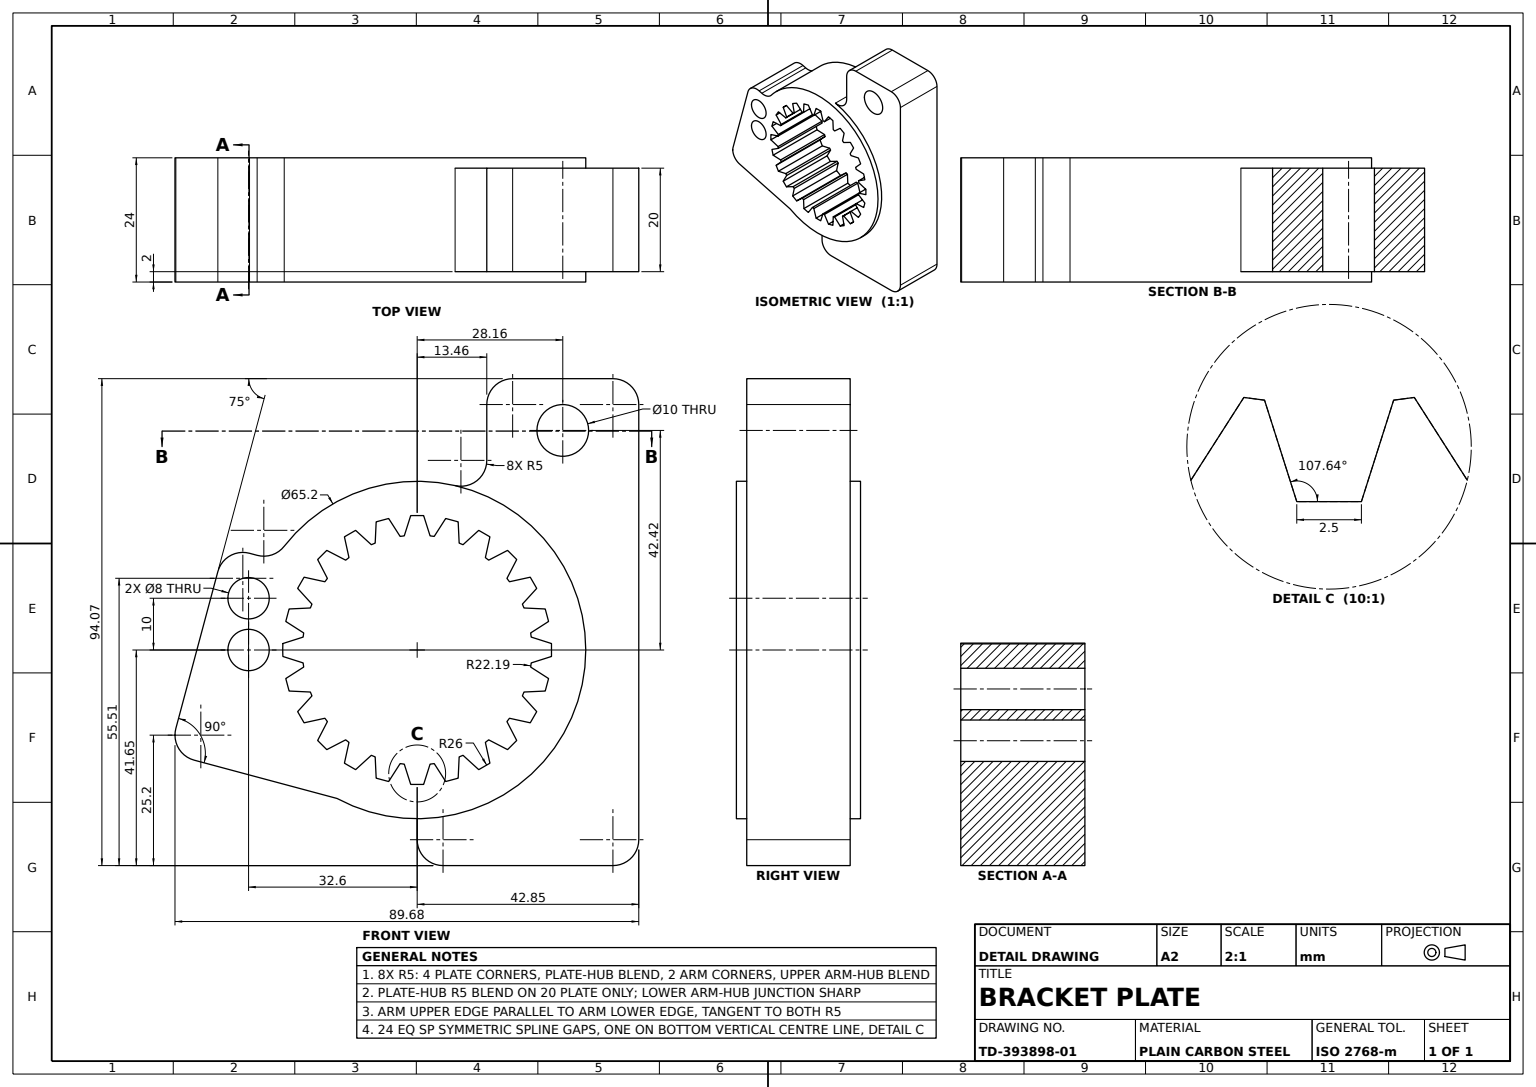
solid
v1 (-20.651843,-8.117725,-12)
v2 (-20.343157,-8.86296,-12)
e1 v1 v2 CIRCLE(AX(P(0,0,-12),D(0,0,1),D(1,0,0)),22.19)
v3 (-20.651843,-8.117725,12)
e2 v3 v1 LINE
v4 (-20.343157,-8.86296,12)
e3 v3 v4 CIRCLE(AX(P(0,0,12),D(0,0,1),D(1,0,0)),22.19)
e4 v4 v2 LINE
face CYL(AX(P(0,0,12),D(0,0,-1),D(-1,0,0)),22.19) rev [-e1 -e2 e3 e4]
v5 (7.335,31.764096,10)
v6 (0,-32.6,10)
e5 v5 v6 CIRCLE(AX(P(0,0,10),D(0,0,-1),D(1,0,0)),32.6)
v7 (0,-36.65,10)
e6 v6 v7 LINE
v8 (5,-41.65,10)
e7 v7 v8 CIRCLE(AX(P(5,-36.65,10),D(0,0,1),D(-1,0,0)),5)
v9 (37.85,-41.65,10)
e8 v8 v9 LINE
v10 (42.85,-36.65,10)
e9 v9 v10 CIRCLE(AX(P(37.85,-36.65,10),D(0,0,1),D(-1,0,0)),5)
v11 (42.85,47.42,10)
e10 v10 v11 LINE
v12 (37.85,52.42,10)
e11 v11 v12 CIRCLE(AX(P(37.85,47.42,10),D(0,0,1),D(-1,0,0)),5)
v13 (18.46,52.42,10)
e12 v12 v13 LINE
v14 (13.46,47.42,10)
e13 v13 v14 CIRCLE(AX(P(18.46,47.42,10),D(0,0,1),D(-1,0,0)),5)
v15 (13.46,36.63589,10)
e14 v14 v15 LINE
e15 v15 v5 CIRCLE(AX(P(8.46,36.63589,10),D(0,0,-1),D(1,0,0)),5)
v16 (33.155,42.42,10)
v17 (23.155,42.42,10)
e16 v16 v17 CIRCLE(AX(P(28.155,42.42,10),D(0,0,1),D(1,0,0)),5)
e17 v17 v16 CIRCLE(AX(P(28.155,42.42,10),D(0,0,1),D(1,0,0)),5)
face PLANE(AX(P(37.85,-36.65,10),D(0,0,-1),D(-1,0,0))) rev [e5 e6 e7 e8 e9 e10 e11 e12 e13 e14 e15] [-e16 -e17]
v18 (25.408478,5.51446,12)
v19 (25.408478,5.51446,-12)
e18 v18 v19 LINE
v20 (21.943884,3.295765,-12)
e19 v20 v19 LINE
v21 (21.943884,3.295765,12)
e20 v21 v20 LINE
e21 v21 v18 LINE
face PLANE(AX(P(4.885198,-7.628462,12),D(-0.539287232,0.842121892,0),D(-0.842121892,-0.539287232,0))) [e18 -e19 -e20 e21]
v22 (-2.49603,22.049171,12)
v23 (-3.295765,21.943884,12)
e22 v22 v23 CIRCLE(AX(P(0,0,12),D(0,0,1),D(1,0,0)),22.19)
v24 (-3.295765,21.943884,-12)
e23 v23 v24 LINE
v25 (-2.49603,22.049171,-12)
e24 v25 v24 CIRCLE(AX(P(0,0,-12),D(0,0,1),D(1,0,0)),22.19)
e25 v22 v25 LINE
face CYL(AX(P(0,0,12),D(0,0,-1),D(-1,0,0)),22.19) rev [e22 e23 -e24 -e25]
v26 (1.249639,25.969952,12)
v27 (1.249639,25.969952,-12)
e26 v26 v27 LINE
v28 (2.49603,22.049171,-12)
e27 v28 v27 LINE
v29 (2.49603,22.049171,12)
e28 v29 v28 LINE
e29 v29 v26 LINE
face PLANE(AX(P(8.632911,2.744348,12),D(-0.953005091,-0.302954281,0),D(0.302954281,-0.953005091,0))) [e26 -e27 -e28 e29]
v30 (-1.249639,25.969952,-12)
e30 v27 v30 CIRCLE(AX(P(0,0,-12),D(0,0,1),D(1,0,0)),26)
v31 (-1.249639,25.969952,12)
e31 v26 v31 CIRCLE(AX(P(0,0,12),D(0,0,1),D(1,0,0)),26)
e32 v31 v30 LINE
face CYL(AX(P(0,0,12),D(0,0,-1),D(-1,0,0)),26) rev [-e30 -e26 e31 e32]
v32 (-21.865819,14.067195,12)
v33 (-21.865819,14.067195,-12)
e33 v32 v33 LINE
v34 (-17.847127,13.186211,-12)
e34 v34 v33 LINE
v35 (-17.847127,13.186211,12)
e35 v35 v34 LINE
e36 v35 v32 LINE
face PLANE(AX(P(1.939781,8.848494,12),D(-0.214136442,-0.976803759,0),D(0.976803759,-0.214136442,0))) [e33 -e34 -e35 e36]
v36 (20.343157,-8.86296,12)
v37 (20.651843,-8.117725,12)
e37 v36 v37 CIRCLE(AX(P(0,0,12),D(0,0,1),D(1,0,0)),22.19)
v38 (20.651843,-8.117725,-12)
e38 v37 v38 LINE
v39 (20.343157,-8.86296,-12)
e39 v39 v38 CIRCLE(AX(P(0,0,-12),D(0,0,1),D(1,0,0)),22.19)
e40 v36 v39 LINE
face CYL(AX(P(0,0,12),D(0,0,-1),D(-1,0,0)),22.19) rev [e37 e38 -e39 -e40]
v40 (33.155,42.42,-10)
e41 v40 v16 LINE
v41 (23.155,42.42,-10)
e42 v41 v40 CIRCLE(AX(P(28.155,42.42,-10),D(0,0,1),D(1,0,0)),5)
e43 v41 v17 LINE
face CYL(AX(P(28.155,42.42,-10),D(0,0,1),D(1,0,0)),5) rev [e17 -e41 -e42 e43]
v42 (-26,0,12)
v43 (-26,0,-12)
e44 v42 v43 LINE
v44 (-25.969952,1.249639,-12)
e45 v44 v43 CIRCLE(AX(P(0,0,-12),D(0,0,1),D(1,0,0)),26)
v45 (-25.969952,1.249639,12)
e46 v45 v44 LINE
e47 v45 v42 CIRCLE(AX(P(0,0,12),D(0,0,1),D(1,0,0)),26)
face CYL(AX(P(0,0,12),D(0,0,-1),D(-1,0,0)),26) rev [e44 -e45 -e46 e47]
v46 (-17.356078,13.826158,12)
e48 v46 v35 CIRCLE(AX(P(0,0,12),D(0,0,1),D(1,0,0)),22.19)
v47 (-17.356078,13.826158,-12)
e49 v47 v34 CIRCLE(AX(P(0,0,-12),D(0,0,1),D(1,0,0)),22.19)
e50 v46 v47 LINE
face CYL(AX(P(0,0,12),D(0,0,-1),D(-1,0,0)),22.19) rev [e48 e35 -e49 -e50]
v48 (-43.125337,-21.279101,-12)
v49 (-15.4932,-28.683109,-12)
e51 v48 v49 LINE
v50 (-15.4932,-28.683109,12)
e52 v50 v49 LINE
v51 (-43.125337,-21.279101,12)
e53 v51 v50 LINE
e54 v51 v48 LINE
face PLANE(AX(P(-47.954966,-19.985005,12),D(0.258819045,0.965925826,0),D(-0.965925826,0.258819045,0))) rev [e51 -e52 -e53 e54]
v52 (-38.540423,15.150547,-12)
v53 (-46.660871,-15.155376,-12)
e55 v52 v53 LINE
v54 (-46.660871,-15.155376,12)
e56 v53 v54 LINE
v55 (-38.540423,15.150547,12)
e57 v55 v54 LINE
e58 v55 v52 LINE
face PLANE(AX(P(-37.246328,19.980176,12),D(0.965925826,-0.258819045,0),D(0.258819045,0.965925826,0))) rev [e55 e56 -e57 e58]
v56 (25.408478,-5.51446,12)
v57 (25.408478,-5.51446,-12)
e59 v56 v57 LINE
v58 (21.943884,-3.295765,12)
e60 v58 v56 LINE
v59 (21.943884,-3.295765,-12)
e61 v58 v59 LINE
e62 v59 v57 LINE
face PLANE(AX(P(4.885198,7.628462,12),D(0.539287232,0.842121892,0),D(-0.842121892,0.539287232,0))) rev [-e59 -e60 e61 e62]
v60 (-46.831242,-16.449471,12)
v61 (-46.831242,-16.449471,-12)
e63 v60 v61 LINE
e64 v54 v60 CIRCLE(AX(P(-41.831242,-16.449471,12),D(0,0,1),D(1,0,0)),5)
e65 v61 v53 CIRCLE(AX(P(-41.831242,-16.449471,-12),D(0,0,-1),D(1,0,0)),5)
face CYL(AX(P(-41.831242,-16.449471,12),D(0,0,-1),D(-1,0,0)),5) [-e63 -e64 -e56 -e65]
v62 (3.295765,-21.943884,12)
v63 (3.295765,-21.943884,-12)
e66 v62 v63 LINE
v64 (2.49603,-22.049171,-12)
e67 v64 v63 CIRCLE(AX(P(0,0,-12),D(0,0,1),D(1,0,0)),22.19)
v65 (2.49603,-22.049171,12)
e68 v65 v64 LINE
e69 v65 v62 CIRCLE(AX(P(0,0,12),D(0,0,1),D(1,0,0)),22.19)
face CYL(AX(P(0,0,12),D(0,0,-1),D(-1,0,0)),22.19) rev [e66 -e67 -e68 e69]
v66 (8.86296,20.343157,-12)
v67 (11.902757,23.115457,-12)
e70 v66 v67 LINE
v68 (11.902757,23.115457,12)
e71 v68 v67 LINE
v69 (8.86296,20.343157,12)
e72 v69 v68 LINE
e73 v69 v66 LINE
face PLANE(AX(P(-6.104147,6.693131,12),D(-0.673849478,0.738868649,0),D(-0.738868649,-0.673849478,0))) rev [e70 -e71 -e72 e73]
v70 (20.343157,8.86296,12)
v71 (20.343157,8.86296,-12)
e74 v70 v71 LINE
v72 (23.115457,11.902757,12)
e75 v70 v72 LINE
v73 (23.115457,11.902757,-12)
e76 v72 v73 LINE
e77 v71 v73 LINE
face PLANE(AX(P(6.693131,-6.104147,12),D(-0.738868649,0.673849478,0),D(-0.673849478,-0.738868649,0))) [-e74 e75 e76 -e77]
v74 (-1.249639,-25.969952,12)
v75 (1.249639,-25.969952,12)
e78 v74 v75 CIRCLE(AX(P(0,0,12),D(0,0,1),D(1,0,0)),26)
v76 (1.249639,-25.969952,-12)
e79 v75 v76 LINE
v77 (-1.249639,-25.969952,-12)
e80 v77 v76 CIRCLE(AX(P(0,0,-12),D(0,0,1),D(1,0,0)),26)
e81 v74 v77 LINE
face CYL(AX(P(0,0,12),D(0,0,-1),D(-1,0,0)),26) rev [e78 e79 -e80 -e81]
v78 (37.85,-41.65,-10)
e82 v9 v78 LINE
v79 (42.85,-36.65,-10)
e83 v78 v79 CIRCLE(AX(P(37.85,-36.65,-10),D(0,0,1),D(-1,0,0)),5)
e84 v10 v79 LINE
face CYL(AX(P(37.85,-36.65,10),D(0,0,-1),D(-1,0,0)),5) [e82 e83 -e84 -e9]
v80 (-14.067195,-21.865819,12)
v81 (-14.067195,-21.865819,-12)
e85 v80 v81 LINE
v82 (-11.902757,-23.115457,12)
e86 v80 v82 CIRCLE(AX(P(0,0,12),D(0,0,1),D(1,0,0)),26)
v83 (-11.902757,-23.115457,-12)
e87 v82 v83 LINE
e88 v81 v83 CIRCLE(AX(P(0,0,-12),D(0,0,1),D(1,0,0)),26)
face CYL(AX(P(0,0,12),D(0,0,-1),D(-1,0,0)),26) rev [-e85 e86 e87 -e88]
v84 (-24.761617,-7.928577,-12)
e89 v1 v84 LINE
v85 (-24.761617,-7.928577,12)
e90 v85 v84 LINE
e91 v3 v85 LINE
face PLANE(AX(P(-0.416475,-9.049041,12),D(-0.045975497,-0.998942568,0),D(0.998942568,-0.045975497,0))) rev [e89 -e90 -e91 e2]
v86 (18.46,52.42,-10)
v87 (13.46,47.42,-10)
e92 v86 v87 CIRCLE(AX(P(18.46,47.42,-10),D(0,0,1),D(-1,0,0)),5)
e93 v14 v87 LINE
e94 v13 v86 LINE
face CYL(AX(P(18.46,47.42,10),D(0,0,-1),D(-1,0,0)),5) [e92 -e93 -e13 e94]
v88 (13.186211,-17.847127,-12)
v89 (13.826158,-17.356078,-12)
e95 v88 v89 CIRCLE(AX(P(0,0,-12),D(0,0,1),D(1,0,0)),22.19)
v90 (13.186211,-17.847127,12)
e96 v90 v88 LINE
v91 (13.826158,-17.356078,12)
e97 v90 v91 CIRCLE(AX(P(0,0,12),D(0,0,1),D(1,0,0)),22.19)
e98 v91 v89 LINE
face CYL(AX(P(0,0,12),D(0,0,-1),D(-1,0,0)),22.19) rev [-e95 -e96 e97 e98]
v92 (37.85,52.42,-10)
e99 v92 v86 LINE
e100 v12 v92 LINE
face PLANE(AX(P(37.85,52.42,10),D(0,-1,0),D(0,0,-1))) rev [e99 -e94 -e12 e100]
v93 (-28.6,10,-12)
v94 (-28.6,10,12)
e101 v93 v94 LINE
v95 (-36.6,10,12)
e102 v94 v95 CIRCLE(AX(P(-32.6,10,12),D(0,0,1),D(1,0,0)),4)
v96 (-36.6,10,-12)
e103 v96 v95 LINE
e104 v93 v96 CIRCLE(AX(P(-32.6,10,-12),D(0,0,1),D(1,0,0)),4)
face CYL(AX(P(-32.6,10,-12),D(0,0,1),D(1,0,0)),4) rev [e101 e102 -e103 -e104]
v97 (-17.847127,-13.186211,12)
v98 (-21.865819,-14.067195,12)
e105 v97 v98 LINE
v99 (-17.847127,-13.186211,-12)
e106 v97 v99 LINE
v100 (-21.865819,-14.067195,-12)
e107 v99 v100 LINE
e108 v98 v100 LINE
face PLANE(AX(P(1.939781,-8.848494,12),D(0.214136442,-0.976803759,0),D(0.976803759,0.214136442,0))) rev [-e105 e106 e107 -e108]
v101 (17.356078,-13.826158,12)
v102 (17.356078,-13.826158,-12)
e109 v101 v102 LINE
v103 (17.847127,-13.186211,12)
e110 v101 v103 CIRCLE(AX(P(0,0,12),D(0,0,1),D(1,0,0)),22.19)
v104 (17.847127,-13.186211,-12)
e111 v103 v104 LINE
e112 v102 v104 CIRCLE(AX(P(0,0,-12),D(0,0,1),D(1,0,0)),22.19)
face CYL(AX(P(0,0,12),D(0,0,-1),D(-1,0,0)),22.19) rev [-e109 e110 e111 -e112]
v105 (-23.115457,11.902757,12)
e113 v32 v105 CIRCLE(AX(P(0,0,12),D(0,0,1),D(1,0,0)),26)
v106 (-23.115457,11.902757,-12)
e114 v105 v106 LINE
e115 v33 v106 CIRCLE(AX(P(0,0,-12),D(0,0,1),D(1,0,0)),26)
face CYL(AX(P(0,0,12),D(0,0,-1),D(-1,0,0)),26) rev [-e33 e113 e114 -e115]
v107 (-17.356078,-13.826158,12)
v108 (-19.247157,-17.479901,12)
e116 v107 v108 LINE
v109 (-19.247157,-17.479901,-12)
e117 v108 v109 LINE
v110 (-17.356078,-13.826158,-12)
e118 v110 v109 LINE
e119 v107 v110 LINE
face PLANE(AX(P(-8.044937,4.163843,12),D(0.888097389,-0.459655336,0),D(0.459655336,0.888097389,0))) [e116 e117 -e118 -e119]
v111 (19.247157,-17.479901,12)
v112 (19.247157,-17.479901,-12)
e120 v111 v112 LINE
e121 v101 v111 LINE
e122 v102 v112 LINE
face PLANE(AX(P(8.044937,4.163843,12),D(0.888097389,0.459655336,0),D(-0.459655336,0.888097389,0))) rev [-e120 -e121 e109 e122]
v113 (23.115457,-11.902757,-12)
e123 v39 v113 LINE
v114 (23.115457,-11.902757,12)
e124 v114 v113 LINE
e125 v36 v114 LINE
face PLANE(AX(P(6.693131,6.104147,12),D(0.738868649,0.673849478,0),D(-0.673849478,0.738868649,0))) rev [e40 e123 -e124 -e125]
v115 (14.067195,-21.865819,12)
v116 (14.067195,-21.865819,-12)
e126 v115 v116 LINE
v117 (11.902757,-23.115457,-12)
e127 v117 v116 CIRCLE(AX(P(0,0,-12),D(0,0,1),D(1,0,0)),26)
v118 (11.902757,-23.115457,12)
e128 v118 v117 LINE
e129 v118 v115 CIRCLE(AX(P(0,0,12),D(0,0,1),D(1,0,0)),26)
face CYL(AX(P(0,0,12),D(0,0,-1),D(-1,0,0)),26) rev [e126 -e127 -e128 e129]
v119 (8.86296,-20.343157,12)
v120 (8.86296,-20.343157,-12)
e130 v119 v120 LINE
v121 (8.117725,-20.651843,-12)
e131 v121 v120 CIRCLE(AX(P(0,0,-12),D(0,0,1),D(1,0,0)),22.19)
v122 (8.117725,-20.651843,12)
e132 v122 v121 LINE
e133 v122 v119 CIRCLE(AX(P(0,0,12),D(0,0,1),D(1,0,0)),22.19)
face CYL(AX(P(0,0,12),D(0,0,-1),D(-1,0,0)),22.19) rev [e130 -e131 -e132 e133]
v123 (17.847127,13.186211,12)
v124 (17.356078,13.826158,12)
e134 v123 v124 CIRCLE(AX(P(0,0,12),D(0,0,1),D(1,0,0)),22.19)
v125 (17.356078,13.826158,-12)
e135 v124 v125 LINE
v126 (17.847127,13.186211,-12)
e136 v126 v125 CIRCLE(AX(P(0,0,-12),D(0,0,1),D(1,0,0)),22.19)
e137 v123 v126 LINE
face CYL(AX(P(0,0,12),D(0,0,-1),D(-1,0,0)),22.19) rev [e134 e135 -e136 -e137]
v127 (5,-41.65,-10)
e138 v127 v78 LINE
v128 (0,-36.65,-10)
e139 v128 v127 CIRCLE(AX(P(5,-36.65,-10),D(0,0,1),D(-1,0,0)),5)
v129 (0,-32.6,-10)
e140 v129 v128 LINE
v130 (7.335,31.764096,-10)
e141 v130 v129 CIRCLE(AX(P(0,0,-10),D(0,0,-1),D(1,0,0)),32.6)
v131 (13.46,36.63589,-10)
e142 v131 v130 CIRCLE(AX(P(8.46,36.63589,-10),D(0,0,-1),D(1,0,0)),5)
e143 v87 v131 LINE
v132 (42.85,47.42,-10)
e144 v132 v92 CIRCLE(AX(P(37.85,47.42,-10),D(0,0,1),D(-1,0,0)),5)
e145 v79 v132 LINE
e146 v40 v41 CIRCLE(AX(P(28.155,42.42,-10),D(0,0,1),D(1,0,0)),5)
face PLANE(AX(P(37.85,-36.65,-10),D(0,0,-1),D(-1,0,0))) [-e83 -e138 -e139 -e140 -e141 -e142 -e143 -e92 -e99 -e144 -e145] [e42 e146]
v133 (14.067195,21.865819,-12)
e147 v133 v67 CIRCLE(AX(P(0,0,-12),D(0,0,1),D(1,0,0)),26)
v134 (14.067195,21.865819,12)
e148 v134 v133 LINE
e149 v134 v68 CIRCLE(AX(P(0,0,12),D(0,0,1),D(1,0,0)),26)
face CYL(AX(P(0,0,12),D(0,0,-1),D(-1,0,0)),26) rev [e71 -e147 -e148 e149]
v135 (21.865819,14.067195,12)
e150 v123 v135 LINE
v136 (21.865819,14.067195,-12)
e151 v126 v136 LINE
e152 v135 v136 LINE
face PLANE(AX(P(-1.939781,8.848494,12),D(-0.214136442,0.976803759,0),D(-0.976803759,-0.214136442,0))) rev [-e150 e137 e151 -e152]
v137 (5.51446,-25.408478,12)
v138 (7.928577,-24.761617,12)
e153 v137 v138 CIRCLE(AX(P(0,0,12),D(0,0,1),D(1,0,0)),26)
v139 (7.928577,-24.761617,-12)
e154 v138 v139 LINE
v140 (5.51446,-25.408478,-12)
e155 v140 v139 CIRCLE(AX(P(0,0,-12),D(0,0,1),D(1,0,0)),26)
e156 v137 v140 LINE
face CYL(AX(P(0,0,12),D(0,0,-1),D(-1,0,0)),26) rev [e153 e154 -e155 -e156]
v141 (13.826158,17.356078,-12)
v142 (13.186211,17.847127,-12)
e157 v141 v142 CIRCLE(AX(P(0,0,-12),D(0,0,1),D(1,0,0)),22.19)
v143 (13.826158,17.356078,12)
e158 v143 v141 LINE
v144 (13.186211,17.847127,12)
e159 v143 v144 CIRCLE(AX(P(0,0,12),D(0,0,1),D(1,0,0)),22.19)
e160 v144 v142 LINE
face CYL(AX(P(0,0,12),D(0,0,-1),D(-1,0,0)),22.19) rev [-e157 -e158 e159 e160]
v145 (19.247157,17.479901,12)
v146 (19.247157,17.479901,-12)
e161 v145 v146 LINE
v147 (17.479901,19.247157,12)
e162 v145 v147 CIRCLE(AX(P(0,0,12),D(0,0,1),D(1,0,0)),26)
v148 (17.479901,19.247157,-12)
e163 v147 v148 LINE
e164 v146 v148 CIRCLE(AX(P(0,0,-12),D(0,0,1),D(1,0,0)),26)
face CYL(AX(P(0,0,12),D(0,0,-1),D(-1,0,0)),26) rev [-e161 e162 e163 -e164]
v149 (-17.479901,19.247157,12)
v150 (-19.247157,17.479901,12)
e165 v149 v150 CIRCLE(AX(P(0,0,12),D(0,0,1),D(1,0,0)),26)
v151 (-19.247157,17.479901,-12)
e166 v150 v151 LINE
v152 (-17.479901,19.247157,-12)
e167 v152 v151 CIRCLE(AX(P(0,0,-12),D(0,0,1),D(1,0,0)),26)
e168 v149 v152 LINE
face CYL(AX(P(0,0,12),D(0,0,-1),D(-1,0,0)),26) rev [e165 e166 -e167 -e168]
v153 (22.049171,2.49603,-12)
e169 v153 v20 CIRCLE(AX(P(0,0,-12),D(0,0,1),D(1,0,0)),22.19)
v154 (22.049171,2.49603,12)
e170 v154 v153 LINE
e171 v154 v21 CIRCLE(AX(P(0,0,12),D(0,0,1),D(1,0,0)),22.19)
face CYL(AX(P(0,0,12),D(0,0,-1),D(-1,0,0)),22.19) rev [e20 -e169 -e170 e171]
v155 (-21.943884,3.295765,-12)
v156 (-25.408478,5.51446,-12)
e172 v155 v156 LINE
v157 (-25.408478,5.51446,12)
e173 v157 v156 LINE
v158 (-21.943884,3.295765,12)
e174 v158 v157 LINE
e175 v158 v155 LINE
face PLANE(AX(P(-4.885198,-7.628462,12),D(-0.539287232,-0.842121892,0),D(0.842121892,-0.539287232,0))) rev [e172 -e173 -e174 e175]
v159 (20.651843,8.117725,12)
e176 v159 v70 CIRCLE(AX(P(0,0,12),D(0,0,1),D(1,0,0)),22.19)
v160 (20.651843,8.117725,-12)
e177 v160 v71 CIRCLE(AX(P(0,0,-12),D(0,0,1),D(1,0,0)),22.19)
e178 v159 v160 LINE
face CYL(AX(P(0,0,12),D(0,0,-1),D(-1,0,0)),22.19) rev [e176 e74 -e177 -e178]
v161 (-25.969952,-1.249639,12)
e179 v42 v161 CIRCLE(AX(P(0,0,12),D(0,0,1),D(1,0,0)),26)
v162 (-25.969952,-1.249639,-12)
e180 v161 v162 LINE
e181 v43 v162 CIRCLE(AX(P(0,0,-12),D(0,0,1),D(1,0,0)),26)
face CYL(AX(P(0,0,12),D(0,0,-1),D(-1,0,0)),26) rev [-e44 e179 e180 -e181]
e182 v8 v127 LINE
face PLANE(AX(P(37.85,-41.65,10),D(0,1,0),D(0,0,1))) rev [-e82 -e8 e182 e138]
v163 (-23.115457,-11.902757,12)
e183 v4 v163 LINE
v164 (-23.115457,-11.902757,-12)
e184 v163 v164 LINE
e185 v2 v164 LINE
face PLANE(AX(P(-6.693131,6.104147,12),D(0.738868649,-0.673849478,0),D(0.673849478,0.738868649,0))) [-e4 e183 e184 -e185]
e186 v144 v134 LINE
e187 v142 v133 LINE
face PLANE(AX(P(8.848494,-1.939781,12),D(-0.976803759,0.214136442,0),D(-0.214136442,-0.976803759,0))) [e186 e148 -e187 -e160]
v165 (24.761617,-7.928577,-12)
e188 v165 v57 CIRCLE(AX(P(0,0,-12),D(0,0,1),D(1,0,0)),26)
v166 (24.761617,-7.928577,12)
e189 v166 v165 LINE
e190 v166 v56 CIRCLE(AX(P(0,0,12),D(0,0,1),D(1,0,0)),26)
face CYL(AX(P(0,0,12),D(0,0,-1),D(-1,0,0)),26) rev [e59 -e188 -e189 e190]
v167 (-25.707798,20.046674,12)
v168 (-30.944807,18.291688,12)
e191 v167 v168 CIRCLE(AX(P(-29.650711,23.121317,12),D(0,0,-1),D(1,0,0)),5)
v169 (-25.707798,20.046674,-12)
e192 v169 v167 LINE
v170 (-30.944807,18.291688,-12)
e193 v170 v169 CIRCLE(AX(P(-29.650711,23.121317,-12),D(0,0,1),D(1,0,0)),5)
e194 v168 v170 LINE
face CYL(AX(P(-29.650711,23.121317,12),D(0,0,-1),D(-1,0,0)),5) rev [-e191 -e192 -e193 -e194]
e195 v11 v132 LINE
face CYL(AX(P(37.85,47.42,10),D(0,0,-1),D(-1,0,0)),5) [-e100 -e11 e195 e144]
v171 (-2.49603,-22.049171,12)
v172 (-2.49603,-22.049171,-12)
e196 v171 v172 LINE
e197 v171 v74 LINE
e198 v172 v77 LINE
face PLANE(AX(P(-8.632911,-2.744348,12),D(0.953005091,0.302954281,0),D(-0.302954281,0.953005091,0))) [-e196 e197 e81 -e198]
v173 (22.049171,-2.49603,-12)
e199 v59 v173 CIRCLE(AX(P(0,0,-12),D(0,0,1),D(1,0,0)),22.19)
v174 (22.049171,-2.49603,12)
e200 v58 v174 CIRCLE(AX(P(0,0,12),D(0,0,1),D(1,0,0)),22.19)
e201 v174 v173 LINE
face CYL(AX(P(0,0,12),D(0,0,-1),D(-1,0,0)),22.19) rev [-e199 -e61 e200 e201]
v175 (7.928577,24.761617,-12)
v176 (5.51446,25.408478,-12)
e202 v175 v176 CIRCLE(AX(P(0,0,-12),D(0,0,1),D(1,0,0)),26)
v177 (7.928577,24.761617,12)
e203 v177 v175 LINE
v178 (5.51446,25.408478,12)
e204 v177 v178 CIRCLE(AX(P(0,0,12),D(0,0,1),D(1,0,0)),26)
e205 v178 v176 LINE
face CYL(AX(P(0,0,12),D(0,0,-1),D(-1,0,0)),26) rev [-e202 -e203 e204 e205]
v179 (-13.186211,17.847127,12)
v180 (-13.826158,17.356078,12)
e206 v179 v180 CIRCLE(AX(P(0,0,12),D(0,0,1),D(1,0,0)),22.19)
v181 (-13.826158,17.356078,-12)
e207 v180 v181 LINE
v182 (-13.186211,17.847127,-12)
e208 v182 v181 CIRCLE(AX(P(0,0,-12),D(0,0,1),D(1,0,0)),22.19)
e209 v179 v182 LINE
face CYL(AX(P(0,0,12),D(0,0,-1),D(-1,0,0)),22.19) rev [e206 e207 -e208 -e209]
v183 (-3.295765,-21.943884,12)
v184 (-5.51446,-25.408478,12)
e210 v183 v184 LINE
v185 (-3.295765,-21.943884,-12)
e211 v183 v185 LINE
v186 (-5.51446,-25.408478,-12)
e212 v185 v186 LINE
e213 v184 v186 LINE
face PLANE(AX(P(7.628462,-4.885198,12),D(0.842121892,-0.539287232,0),D(0.539287232,0.842121892,0))) rev [-e210 e211 e212 -e213]
v187 (-13.186211,-17.847127,12)
e214 v187 v80 LINE
v188 (-13.186211,-17.847127,-12)
e215 v188 v81 LINE
e216 v187 v188 LINE
face PLANE(AX(P(-8.848494,1.939781,12),D(0.976803759,-0.214136442,0),D(0.214136442,0.976803759,0))) [e214 e85 -e215 -e216]
e217 v141 v148 LINE
e218 v143 v147 LINE
face PLANE(AX(P(-4.163843,8.044937,12),D(-0.459655336,0.888097389,0),D(-0.888097389,-0.459655336,0))) rev [e158 e217 -e163 -e218]
v189 (25.969952,1.249639,12)
v190 (25.969952,1.249639,-12)
e219 v189 v190 LINE
e220 v154 v189 LINE
e221 v153 v190 LINE
face PLANE(AX(P(2.744348,8.632911,12),D(0.302954281,0.953005091,0),D(-0.953005091,0.302954281,0))) rev [-e219 -e220 e170 e221]
e222 v65 v75 LINE
e223 v64 v76 LINE
face PLANE(AX(P(8.632911,-2.744348,12),D(0.953005091,-0.302954281,0),D(0.302954281,0.953005091,0))) rev [-e222 e68 e223 -e79]
v191 (-8.86296,20.343157,-12)
v192 (-11.902757,23.115457,-12)
e224 v191 v192 LINE
v193 (-8.86296,20.343157,12)
e225 v193 v191 LINE
v194 (-11.902757,23.115457,12)
e226 v193 v194 LINE
e227 v194 v192 LINE
face PLANE(AX(P(6.104147,6.693131,12),D(-0.673849478,-0.738868649,0),D(0.738868649,-0.673849478,0))) [-e224 -e225 e226 e227]
v195 (-22.049171,2.49603,-12)
e228 v195 v44 LINE
v196 (-22.049171,2.49603,12)
e229 v196 v195 LINE
e230 v196 v45 LINE
face PLANE(AX(P(-2.744348,8.632911,12),D(0.302954281,-0.953005091,0),D(0.953005091,0.302954281,0))) [e46 -e228 -e229 e230]
v197 (8.117725,20.651843,-12)
e231 v66 v197 CIRCLE(AX(P(0,0,-12),D(0,0,1),D(1,0,0)),22.19)
v198 (8.117725,20.651843,12)
e232 v69 v198 CIRCLE(AX(P(0,0,12),D(0,0,1),D(1,0,0)),22.19)
e233 v198 v197 LINE
face CYL(AX(P(0,0,12),D(0,0,-1),D(-1,0,0)),22.19) rev [-e231 -e73 e232 e233]
v199 (-17.479901,-19.247157,12)
v200 (-17.479901,-19.247157,-12)
e234 v199 v200 LINE
v201 (-13.826158,-17.356078,12)
e235 v201 v199 LINE
v202 (-13.826158,-17.356078,-12)
e236 v201 v202 LINE
e237 v202 v200 LINE
face PLANE(AX(P(4.163843,-8.044937,12),D(0.459655336,-0.888097389,0),D(0.888097389,0.459655336,0))) rev [-e234 -e235 e236 e237]
e238 v7 v128 LINE
e239 v6 v129 LINE
face PLANE(AX(P(0,-36.65,10),D(1,0,0),D(0,0,-1))) rev [-e238 -e6 e239 e140]
v203 (21.865819,-14.067195,12)
v204 (21.865819,-14.067195,-12)
e240 v203 v204 LINE
e241 v203 v114 CIRCLE(AX(P(0,0,12),D(0,0,1),D(1,0,0)),26)
e242 v204 v113 CIRCLE(AX(P(0,0,-12),D(0,0,1),D(1,0,0)),26)
face CYL(AX(P(0,0,12),D(0,0,-1),D(-1,0,0)),26) rev [-e240 e241 e124 -e242]
e243 v60 v51 CIRCLE(AX(P(-41.831242,-16.449471,12),D(0,0,1),D(1,0,0)),5)
e244 v48 v61 CIRCLE(AX(P(-41.831242,-16.449471,-12),D(0,0,-1),D(1,0,0)),5)
face CYL(AX(P(-41.831242,-16.449471,12),D(0,0,-1),D(-1,0,0)),5) [-e54 -e243 e63 -e244]
v205 (-36.6,0,-12)
v206 (-36.6,0,12)
e245 v205 v206 LINE
v207 (-28.6,0,-12)
e246 v207 v205 CIRCLE(AX(P(-32.6,0,-12),D(0,0,1),D(1,0,0)),4)
v208 (-28.6,0,12)
e247 v207 v208 LINE
e248 v208 v206 CIRCLE(AX(P(-32.6,0,12),D(0,0,1),D(1,0,0)),4)
face CYL(AX(P(-32.6,0,-12),D(0,0,1),D(1,0,0)),4) rev [-e245 -e246 e247 e248]
e249 v180 v149 LINE
e250 v181 v152 LINE
face PLANE(AX(P(4.163843,8.044937,12),D(-0.459655336,-0.888097389,0),D(0.888097389,-0.459655336,0))) [e249 e168 -e250 -e207]
v209 (-5.51446,25.408478,12)
v210 (-7.928577,24.761617,12)
e251 v209 v210 CIRCLE(AX(P(0,0,12),D(0,0,1),D(1,0,0)),26)
v211 (-7.928577,24.761617,-12)
e252 v210 v211 LINE
v212 (-5.51446,25.408478,-12)
e253 v212 v211 CIRCLE(AX(P(0,0,-12),D(0,0,1),D(1,0,0)),26)
e254 v209 v212 LINE
face CYL(AX(P(0,0,12),D(0,0,-1),D(-1,0,0)),26) rev [e251 e252 -e253 -e254]
e255 v104 v204 LINE
e256 v103 v203 LINE
face PLANE(AX(P(-1.939781,-8.848494,12),D(0.214136442,0.976803759,0),D(-0.976803759,0.214136442,0))) [-e255 -e111 e256 e240]
e257 v108 v199 CIRCLE(AX(P(0,0,12),D(0,0,1),D(1,0,0)),26)
e258 v109 v200 CIRCLE(AX(P(0,0,-12),D(0,0,1),D(1,0,0)),26)
face CYL(AX(P(0,0,12),D(0,0,-1),D(-1,0,0)),26) rev [e257 e234 -e258 -e117]
face CYL(AX(P(28.155,42.42,-10),D(0,0,1),D(1,0,0)),5) rev [e16 -e43 -e146 e41]
e259 v90 v115 LINE
e260 v88 v116 LINE
face PLANE(AX(P(8.848494,1.939781,12),D(0.976803759,0.214136442,0),D(-0.214136442,0.976803759,0))) rev [-e126 -e259 e96 e260]
v213 (-14.067195,21.865819,12)
e261 v179 v213 LINE
v214 (-14.067195,21.865819,-12)
e262 v182 v214 LINE
e263 v213 v214 LINE
face PLANE(AX(P(-8.848494,-1.939781,12),D(-0.976803759,-0.214136442,0),D(0.214136442,-0.976803759,0))) rev [-e261 e209 e262 -e263]
v215 (-7.928577,-24.761617,12)
v216 (-7.928577,-24.761617,-12)
e264 v215 v216 LINE
v217 (-8.117725,-20.651843,-12)
e265 v217 v216 LINE
v218 (-8.117725,-20.651843,12)
e266 v218 v217 LINE
e267 v218 v215 LINE
face PLANE(AX(P(-9.049041,-0.416475,12),D(0.998942568,0.045975497,0),D(-0.045975497,0.998942568,0))) [e264 -e265 -e266 e267]
e268 v62 v137 LINE
e269 v63 v140 LINE
face PLANE(AX(P(-7.628462,-4.885198,12),D(0.842121892,0.539287232,0),D(-0.539287232,0.842121892,0))) [-e66 e268 e156 -e269]
e270 v202 v188 CIRCLE(AX(P(0,0,-12),D(0,0,1),D(1,0,0)),22.19)
e271 v201 v187 CIRCLE(AX(P(0,0,12),D(0,0,1),D(1,0,0)),22.19)
face CYL(AX(P(0,0,12),D(0,0,-1),D(-1,0,0)),22.19) rev [-e270 -e236 e271 e216]
face PLANE(AX(P(42.85,0,10),D(-1,0,0),D(0,0,1))) rev [e84 e145 -e195 -e10]
v219 (-8.86296,-20.343157,12)
e272 v219 v82 LINE
v220 (-8.86296,-20.343157,-12)
e273 v219 v220 LINE
e274 v220 v83 LINE
face PLANE(AX(P(6.104147,-6.693131,12),D(0.673849478,-0.738868649,0),D(0.738868649,0.673849478,0))) rev [-e272 e273 e274 -e87]
v221 (-20.343157,8.86296,12)
v222 (-20.343157,8.86296,-12)
e275 v221 v222 LINE
v223 (-20.651843,8.117725,12)
e276 v221 v223 CIRCLE(AX(P(0,0,12),D(0,0,1),D(1,0,0)),22.19)
v224 (-20.651843,8.117725,-12)
e277 v223 v224 LINE
e278 v222 v224 CIRCLE(AX(P(0,0,-12),D(0,0,1),D(1,0,0)),22.19)
face CYL(AX(P(0,0,12),D(0,0,-1),D(-1,0,0)),22.19) rev [-e275 e276 e277 -e278]
e279 v125 v146 LINE
e280 v124 v145 LINE
face PLANE(AX(P(8.044937,-4.163843,12),D(-0.888097389,0.459655336,0),D(-0.459655336,-0.888097389,0))) [e161 -e279 -e135 e280]
v225 (-8.117725,20.651843,-12)
e281 v225 v191 CIRCLE(AX(P(0,0,-12),D(0,0,1),D(1,0,0)),22.19)
v226 (-8.117725,20.651843,12)
e282 v226 v225 LINE
e283 v226 v193 CIRCLE(AX(P(0,0,12),D(0,0,1),D(1,0,0)),22.19)
face CYL(AX(P(0,0,12),D(0,0,-1),D(-1,0,0)),22.19) rev [-e281 -e282 e283 e225]
e284 v47 v151 LINE
e285 v46 v150 LINE
face PLANE(AX(P(-8.044937,-4.163843,12),D(-0.888097389,-0.459655336,0),D(0.459655336,-0.888097389,0))) rev [e284 -e166 -e285 e50]
e286 v121 v139 LINE
e287 v122 v138 LINE
face PLANE(AX(P(9.049041,-0.416475,12),D(0.998942568,-0.045975497,0),D(0.045975497,0.998942568,0))) rev [e132 e286 -e154 -e287]
e288 v97 v107 CIRCLE(AX(P(0,0,12),D(0,0,1),D(1,0,0)),22.19)
e289 v163 v98 CIRCLE(AX(P(0,0,12),D(0,0,1),D(1,0,0)),26)
v227 (-25.408478,-5.51446,12)
e290 v227 v85 CIRCLE(AX(P(0,0,12),D(0,0,1),D(1,0,0)),26)
v228 (-21.943884,-3.295765,12)
e291 v228 v227 LINE
v229 (-22.049171,-2.49603,12)
e292 v229 v228 CIRCLE(AX(P(0,0,12),D(0,0,1),D(1,0,0)),22.19)
e293 v229 v161 LINE
e294 v158 v196 CIRCLE(AX(P(0,0,12),D(0,0,1),D(1,0,0)),22.19)
v230 (-24.761617,7.928577,12)
e295 v230 v157 CIRCLE(AX(P(0,0,12),D(0,0,1),D(1,0,0)),26)
e296 v223 v230 LINE
e297 v221 v105 LINE
e298 v194 v213 CIRCLE(AX(P(0,0,12),D(0,0,1),D(1,0,0)),26)
e299 v226 v210 LINE
e300 v23 v209 LINE
e301 v22 v31 LINE
v231 (3.295765,21.943884,12)
e302 v231 v29 CIRCLE(AX(P(0,0,12),D(0,0,1),D(1,0,0)),22.19)
e303 v231 v178 LINE
e304 v198 v177 LINE
e305 v72 v135 CIRCLE(AX(P(0,0,12),D(0,0,1),D(1,0,0)),26)
v232 (24.761617,7.928577,12)
e306 v159 v232 LINE
e307 v18 v232 CIRCLE(AX(P(0,0,12),D(0,0,1),D(1,0,0)),26)
v233 (25.969952,-1.249639,12)
e308 v233 v189 CIRCLE(AX(P(0,0,12),D(0,0,1),D(1,0,0)),26)
e309 v174 v233 LINE
e310 v37 v166 LINE
v234 (17.479901,-19.247157,12)
e311 v234 v111 CIRCLE(AX(P(0,0,12),D(0,0,1),D(1,0,0)),26)
e312 v91 v234 LINE
e313 v119 v118 LINE
e314 v183 v171 CIRCLE(AX(P(0,0,12),D(0,0,1),D(1,0,0)),22.19)
e315 v215 v184 CIRCLE(AX(P(0,0,12),D(0,0,1),D(1,0,0)),26)
e316 v219 v218 CIRCLE(AX(P(0,0,12),D(0,0,1),D(1,0,0)),22.19)
e317 v50 v167 CIRCLE(AX(P(0,0,12),D(0,0,1),D(1,0,0)),32.6)
v235 (-32.416699,18.68608,12)
e318 v168 v235 LINE
e319 v235 v55 CIRCLE(AX(P(-33.710794,13.856451,12),D(0,0,1),D(1,0,0)),5)
e320 v95 v94 CIRCLE(AX(P(-32.6,10,12),D(0,0,1),D(1,0,0)),4)
e321 v206 v208 CIRCLE(AX(P(-32.6,0,12),D(0,0,1),D(1,0,0)),4)
face PLANE(AX(P(0,0,12),D(0,0,1),D(1,0,0))) [e235 -e257 -e116 -e288 e105 -e289 -e183 -e3 e91 -e290 -e291 -e292 e293 -e179 -e47 -e230 -e294 e174 -e295 -e296 -e276 e297 -e113 -e36 -e48 e285 -e165 -e249 -e206 e261 -e298 -e226 -e283 e299 -e251 -e300 -e22 e301 -e31 -e29 -e302 e303 -e204 -e304 -e232 e72 -e149 -e186 -e159 e218 -e162 -e280 -e134 e150 -e305 -e75 -e176 e306 -e307 -e21 -e171 e220 -e308 -e309 -e200 e60 -e190 -e310 -e37 e125 -e241 -e256 -e110 e121 -e311 -e312 -e97 e259 -e129 -e313 -e133 e287 -e153 -e268 -e69 e222 -e78 -e197 -e314 e210 -e315 -e267 -e316 e272 -e86 -e214 -e271] [e64 e243 e53 e317 e191 e318 e319 e57] [-e320 -e102] [-e248 -e321]
v236 (-22.049171,-2.49603,-12)
e322 v229 v236 LINE
e323 v236 v162 LINE
face PLANE(AX(P(-2.744348,-8.632911,12),D(-0.302954281,-0.953005091,0),D(0.953005091,-0.302954281,0))) rev [-e293 e322 e323 -e180]
v237 (3.295765,21.943884,-12)
e324 v237 v28 CIRCLE(AX(P(0,0,-12),D(0,0,1),D(1,0,0)),22.19)
e325 v231 v237 LINE
face CYL(AX(P(0,0,12),D(0,0,-1),D(-1,0,0)),22.19) rev [e28 -e324 -e325 e302]
e326 v5 v130 LINE
e327 v49 v169 CIRCLE(AX(P(0,0,-12),D(0,0,1),D(1,0,0)),32.6)
face CYL(AX(P(0,0,12),D(0,0,-1),D(-1,0,0)),32.6) [-e5 e326 e141 -e239] [e52 e327 e192 -e317]
v238 (-21.943884,-3.295765,-12)
e328 v228 v238 LINE
v239 (-25.408478,-5.51446,-12)
e329 v227 v239 LINE
e330 v238 v239 LINE
face PLANE(AX(P(-4.885198,7.628462,12),D(0.539287232,-0.842121892,0),D(0.842121892,0.539287232,0))) [-e328 e291 e329 -e330]
e331 v155 v195 CIRCLE(AX(P(0,0,-12),D(0,0,1),D(1,0,0)),22.19)
face CYL(AX(P(0,0,12),D(0,0,-1),D(-1,0,0)),22.19) rev [e294 e229 -e331 -e175]
v240 (-32.416699,18.68608,-12)
e332 v240 v235 LINE
e333 v52 v240 CIRCLE(AX(P(-33.710794,13.856451,-12),D(0,0,-1),D(1,0,0)),5)
face CYL(AX(P(-33.710794,13.856451,12),D(0,0,-1),D(-1,0,0)),5) [-e319 -e332 -e333 -e58]
e334 v25 v30 LINE
face PLANE(AX(P(-8.632911,2.744348,12),D(-0.953005091,0.302954281,0),D(-0.302954281,-0.953005091,0))) rev [-e301 e25 e334 -e32]
e335 v205 v207 CIRCLE(AX(P(-32.6,0,-12),D(0,0,1),D(1,0,0)),4)
e336 v170 v240 LINE
e337 v96 v93 CIRCLE(AX(P(-32.6,10,-12),D(0,0,1),D(1,0,0)),4)
e338 v24 v212 LINE
e339 v225 v211 LINE
e340 v192 v214 CIRCLE(AX(P(0,0,-12),D(0,0,1),D(1,0,0)),26)
e341 v222 v106 LINE
v241 (-24.761617,7.928577,-12)
e342 v224 v241 LINE
e343 v241 v156 CIRCLE(AX(P(0,0,-12),D(0,0,1),D(1,0,0)),26)
e344 v236 v238 CIRCLE(AX(P(0,0,-12),D(0,0,1),D(1,0,0)),22.19)
e345 v239 v84 CIRCLE(AX(P(0,0,-12),D(0,0,1),D(1,0,0)),26)
e346 v164 v100 CIRCLE(AX(P(0,0,-12),D(0,0,1),D(1,0,0)),26)
e347 v99 v110 CIRCLE(AX(P(0,0,-12),D(0,0,1),D(1,0,0)),22.19)
e348 v220 v217 CIRCLE(AX(P(0,0,-12),D(0,0,1),D(1,0,0)),22.19)
e349 v216 v186 CIRCLE(AX(P(0,0,-12),D(0,0,1),D(1,0,0)),26)
e350 v185 v172 CIRCLE(AX(P(0,0,-12),D(0,0,1),D(1,0,0)),22.19)
e351 v120 v117 LINE
v242 (17.479901,-19.247157,-12)
e352 v89 v242 LINE
e353 v242 v112 CIRCLE(AX(P(0,0,-12),D(0,0,1),D(1,0,0)),26)
e354 v38 v165 LINE
v243 (25.969952,-1.249639,-12)
e355 v173 v243 LINE
e356 v243 v190 CIRCLE(AX(P(0,0,-12),D(0,0,1),D(1,0,0)),26)
v244 (24.761617,7.928577,-12)
e357 v19 v244 CIRCLE(AX(P(0,0,-12),D(0,0,1),D(1,0,0)),26)
e358 v160 v244 LINE
e359 v73 v136 CIRCLE(AX(P(0,0,-12),D(0,0,1),D(1,0,0)),26)
e360 v197 v175 LINE
e361 v237 v176 LINE
face PLANE(AX(P(0,0,-12),D(0,0,1),D(1,0,0))) rev [e246 e335] [e65 -e55 e333 -e336 e193 -e327 -e51 e244] [e337 e104] [e324 e27 e30 -e334 e24 e338 e253 -e339 e281 e224 e340 -e262 e208 e250 e167 -e284 e49 e34 e115 -e341 e278 e342 e343 -e172 e331 e228 e45 e181 -e323 e344 e330 e345 -e89 e1 e185 e346 -e107 e347 e118 e258 -e237 e270 e215 e88 -e274 e348 e265 e349 -e212 e350 e198 e80 -e223 e67 e269 e155 -e286 e131 e351 e127 -e260 e95 e352 e353 -e122 e112 e255 e242 -e123 e39 e354 e188 -e62 e199 e355 e356 -e221 e169 e19 e357 -e358 e177 e77 e359 -e151 e136 e279 e164 -e217 e157 e187 e147 -e70 e231 e360 e202 -e361]
e362 v233 v243 LINE
face PLANE(AX(P(2.744348,-8.632911,12),D(-0.302954281,0.953005091,0),D(-0.953005091,-0.302954281,0))) [e362 -e355 -e201 e309]
face CYL(AX(P(5,-36.65,10),D(0,0,-1),D(-1,0,0)),5) [e238 e139 -e182 -e7]
e363 v234 v242 LINE
face PLANE(AX(P(-4.163843,-8.044937,12),D(0.459655336,0.888097389,0),D(-0.888097389,0.459655336,0))) [-e98 e312 e363 -e352]
face CYL(AX(P(-32.6,10,-12),D(0,0,1),D(1,0,0)),4) rev [-e101 -e337 e103 e320]
face CYL(AX(P(0,0,12),D(0,0,-1),D(-1,0,0)),26) rev [e120 -e353 -e363 e311]
face CYL(AX(P(0,0,12),D(0,0,-1),D(-1,0,0)),26) rev [e315 e213 -e349 -e264]
e364 v232 v244 LINE
face CYL(AX(P(0,0,12),D(0,0,-1),D(-1,0,0)),26) rev [-e357 -e18 e307 e364]
face CYL(AX(P(0,0,12),D(0,0,-1),D(-1,0,0)),22.19) rev [e328 -e344 -e322 e292]
face CYL(AX(P(0,0,12),D(0,0,-1),D(-1,0,0)),26) rev [-e184 e289 e108 -e346]
e365 v230 v241 LINE
face PLANE(AX(P(-0.416475,9.049041,12),D(0.045975497,-0.998942568,0),D(0.998942568,0.045975497,0))) [-e277 e296 e365 -e342]
face CYL(AX(P(0,0,12),D(0,0,-1),D(-1,0,0)),26) rev [-e340 -e227 e298 e263]
face CYL(AX(P(0,0,12),D(0,0,-1),D(-1,0,0)),26) rev [-e365 e295 e173 -e343]
face PLANE(AX(P(0.416475,-9.049041,12),D(-0.045975497,0.998942568,0),D(-0.998942568,-0.045975497,0))) [e189 -e354 -e38 e310]
face CYL(AX(P(0,0,12),D(0,0,-1),D(-1,0,0)),22.19) rev [e119 -e347 -e106 e288]
face CYL(AX(P(0,0,12),D(0,0,-1),D(-1,0,0)),26) rev [e305 e152 -e359 -e76]
face PLANE(AX(P(-37.246328,19.980176,12),D(-0.258819045,-0.965925826,0),D(0.965925826,-0.258819045,0))) rev [e332 -e318 e194 e336]
e366 v15 v131 LINE
face PLANE(AX(P(13.46,47.42,10),D(1,0,0),D(0,0,-1))) rev [-e366 -e14 e93 e143]
face PLANE(AX(P(-7.628462,4.885198,12),D(-0.842121892,0.539287232,0),D(-0.539287232,-0.842121892,0))) rev [e361 -e205 -e303 e325]
face PLANE(AX(P(7.628462,4.885198,12),D(-0.842121892,-0.539287232,0),D(0.539287232,-0.842121892,0))) [-e23 e300 e254 -e338]
face PLANE(AX(P(-9.049041,0.416475,12),D(-0.998942568,0.045975497,0),D(-0.045975497,-0.998942568,0))) rev [-e299 e282 e339 -e252]
face PLANE(AX(P(9.049041,0.416475,12),D(-0.998942568,-0.045975497,0),D(0.045975497,-0.998942568,0))) [e203 -e360 -e233 e304]
face CYL(AX(P(0,0,12),D(0,0,-1),D(-1,0,0)),26) rev [-e356 -e362 e308 e219]
face PLANE(AX(P(-6.104147,-6.693131,12),D(0.673849478,0.738868649,0),D(-0.738868649,0.673849478,0))) [-e351 -e130 e313 e128]
face CYL(AX(P(0,0,12),D(0,0,-1),D(-1,0,0)),26) rev [-e329 e290 e90 -e345]
face CYL(AX(P(-32.6,0,-12),D(0,0,1),D(1,0,0)),4) rev [e245 e321 -e247 -e335]
face PLANE(AX(P(0.416475,9.049041,12),D(0.045975497,0.998942568,0),D(-0.998942568,0.045975497,0))) rev [e178 e358 -e364 -e306]
face CYL(AX(P(0,0,12),D(0,0,-1),D(-1,0,0)),22.19) rev [-e211 e314 e196 -e350]
face CYL(AX(P(8.46,36.63589,10),D(0,0,-1),D(-1,0,0)),5) rev [-e15 e366 e142 -e326]
face PLANE(AX(P(-6.693131,-6.104147,12),D(-0.738868649,-0.673849478,0),D(0.673849478,-0.738868649,0))) rev [-e297 e275 e341 -e114]
face CYL(AX(P(0,0,12),D(0,0,-1),D(-1,0,0)),22.19) rev [e266 -e348 -e273 e316]
